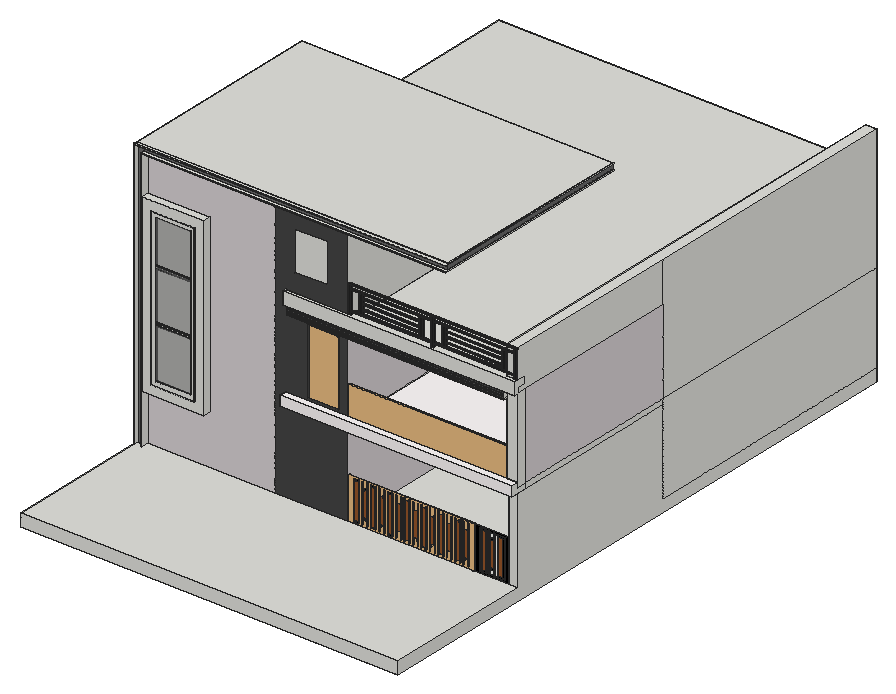
# SketchUp Ruby script. Lengths in inches.
U = 1.inch
M = Sketchup.active_model
def pt(a) = Geom::Point3d.new(a.map { |v| v * U })
def face(e, loops, mat)
  f = e.add_face(loops[0].map { |a| pt(a) })
  loops[1..].each { |l| e.add_face(l.map { |a| pt(a) }).erase! }
  f.material = f.back_material = mat if mat
  f
end
# faces: each face lists its corners as indices into pts; further lists are holes
def faces(e, pts, list, mat = nil) = list.each { |f| face(e, (f[0].is_a?(Array) ? f : [f]).map { |l| l.map { |i| pts[i] } }, mat) }
# xy, xz, yz: faces in a plane at the given z, y or x. An outline is a flat list of corners, or four numbers for a rectangle; further outlines are holes
def ring(l) = l.size == 4 ? [[l[0], l[1]], [l[2], l[1]], [l[2], l[3]], [l[0], l[3]]] : l.each_slice(2).to_a
def flat(e, list, mat, &to3) = list.each { |f| face(e, (f[0].is_a?(Array) ? f : [f]).map { |l| ring(l).map { |u, v| to3.(u, v) } }, mat) }
def xy(e, z, list, mat = nil) = flat(e, list, mat) { |x, y| [x, y, z] }
def xz(e, y, list, mat = nil) = flat(e, list, mat) { |x, z| [x, y, z] }
def yz(e, x, list, mat = nil) = flat(e, list, mat) { |y, z| [x, y, z] }
def lines(e, pts, list) = list.each { |a, b| e.add_line(pt(pts[a]), pt(pts[b])) }
# prism: a flat outline (further loops are holes) pulled along v
def prism(e, loops, v, mat = nil)
  f = face(e, loops, mat); d = Geom::Vector3d.new(v.map { |x| x * U })
  f.pushpull(f.normal.samedirection?(d) ? d.length : -d.length)
end
def box(e, o, s, mat = nil) = prism(e, [[o, [o[0] + s[0], o[1], o[2]], [o[0] + s[0], o[1] + s[1], o[2]], [o[0], o[1] + s[1], o[2]]]], [0, 0, s[2]], mat)
def at(x, y, z, deg = 0) = Geom::Transformation.translation(pt([x, y, z])) * Geom::Transformation.rotation(ORIGIN, Z_AXIS, deg.degrees)
def axes(o, x, y, z) = Geom::Transformation.new([*x, 0, *y, 0, *z, 0, *pt(o).to_a, 1])
def part(name) = M.definitions.add(name)
# library, detail: a bought-in or finely detailed component or shape, given as its bounding box
def library(name, o, s) = part(name).tap { |d| box(d.entities, o, s) }
def detail(e, o, s) = box(e.add_group.entities, o, s)
def put(e, d, t, mat = nil) = e.add_instance(d, t).tap { |i| i.material = mat if mat }
def group(e, t, mat = nil) = e.add_group.tap { |g| g.transformation = t; g.material = mat if mat }.entities
root = M.entities
M.materials.add("Painted Metal Railing").color = [35, 35, 35]
M.materials.add("[0010_Snow]").color = [255, 250, 250]
M.materials.add("[0134_DimGray]").color = [105, 105, 105]
M.materials.add("[0135_DarkGray]").color = [81, 81, 81]
M.materials.add("[Blinds Cellular White]").color = [217, 211, 213]
M.materials.add("[Blinds Cellular White]1").color = [217, 211, 213]
M.materials.add("[Blinds Wood Light]").color = [155, 100, 14]
M.materials.add("[Color M04]").color = [142, 142, 142]
M.materials.add("[Color M09]").color = [0, 0, 0]
M.materials.add("[Granite Dark Gray]").color = [69, 68, 68]
M.materials.add("[Translucent Glass Gray]").color = [128, 128, 128]
M.materials["[Translucent Glass Gray]"].alpha = 0.5
M.materials.add("[Wood Cherry Original]").color = [151, 86, 41]
M.materials.add("[Wood Veneer 01]").color = [119, 70, 35]
c1 = library("Untitled (14)",[0,0,0],[7.13,36,83])
c2 = library("Glass Railings(black Handrails)",[-57.04,-132.55,0],[169.29,2.52,28.17])
c3 = part("Post")
box(c3.entities,[-0.75,-0.75,0],[1.5,1.5,34.5],"Painted Metal Railing")
c4 = part("Group43\#1")
box(c4.entities,[-0.75,0,0],[1.5,73.5,1.5],"Painted Metal Railing")
c5 = part("Group46\#1")
box(c5.entities,[-0.75,0.75,0],[1.5,34.5,1.5],"Painted Metal Railing")
c6 = part("Group49\#1")
box(c6.entities,[-0.75,0.75,0],[1.5,34.5,1.5],"Painted Metal Railing")
c7 = part("Group52\#1")
box(c7.entities,[-0.75,0.75,0],[1.5,34.5,1.5],"Painted Metal Railing")
c8 = part("Group55\#1")
box(c8.entities,[-0.75,0.75,0],[1.5,34.5,1.5],"Painted Metal Railing")
c9 = part("Inner Post")
box(c9.entities,[-0.75,-0.75,0],[1.5,1.5,23.5],"Painted Metal Railing")
c10 = part("Group59\#1")
box(c10.entities,[-0.75,0.75,0],[1.5,24.5,1.5],"Painted Metal Railing")
c11 = part("Group62\#1")
box(c11.entities,[-0.75,0.75,0],[1.5,24.5,1.5],"Painted Metal Railing")
c12 = part("Group65\#1")
box(c12.entities,[-0.75,0.75,0],[1.5,24.5,1.5],"Painted Metal Railing")
c13 = part("Inner Posts and Rails\#2")
put(c13.entities,c9,at(0,0,0,90))
put(c13.entities,c9,at(0,26,0,90))
put(c13.entities,c10,at(0,0,4.75))
put(c13.entities,c11,at(0,0,11))
put(c13.entities,c12,at(0,0,17.25))
c14 = part("Group69\#1")
box(c14.entities,[-0.75,0.75,0],[1.5,24.5,1.5],"Painted Metal Railing")
c15 = part("Group72\#1")
box(c15.entities,[-0.75,0.75,0],[1.5,24.5,1.5],"Painted Metal Railing")
c16 = part("Group75\#1")
box(c16.entities,[-0.75,0.75,0],[1.5,24.5,1.5],"Painted Metal Railing")
c17 = part("Inner Posts and Rails\#3")
put(c17.entities,c9,at(0,0,0,90))
put(c17.entities,c9,at(0,26,0,90))
put(c17.entities,c14,at(0,0,4.75))
put(c17.entities,c15,at(0,0,11))
put(c17.entities,c16,at(0,0,17.25))
c18 = part("Railing Assembly 14\#1")
put(c18.entities,c3,at(0,0,0))
put(c18.entities,c3,at(36,0,0))
put(c18.entities,c3,at(72,0,0))
put(c18.entities,c4,at(-0.75,0,34.5,-90))
put(c18.entities,c5,at(0,0,4,-90))
put(c18.entities,c6,at(36,0,4,-90))
put(c18.entities,c7,at(0,0,29,-90))
put(c18.entities,c8,at(36,0,29,-90))
put(c18.entities,c13,at(5,0,5.5,-90))
put(c18.entities,c17,at(41,0,5.5,-90))
c19 = library("Decorative metal grille",[0,0,0],[271.62,130.55,3])
c20 = part("Group\#1")
xy(c20.entities,0,[[0.39,1.57,0.29,1.59,0.2,1.63,0.12,1.69,0.05,1.77,0.01,1.87,0,1.97,0.01,2.07,0.05,2.17,0.12,2.25,0.2,2.31,0.29,2.35,0.39,2.36,0.5,2.35,0.59,2.31,0.67,2.25,0.73,2.17,0.77,2.07,0.79,1.97,0.77,1.87,0.73,1.77,0.67,1.69,0.59,1.63,0.5,1.59],[0.39,13.39,0.29,13.4,0.2,13.4375,0.12,13.5,0.05,13.58,0.01,13.68,0,13.78,0.01,13.88,0.05,13.98,0.12,14.06,0.2,14.12,0.29,14.16,0.39,14.17,0.5,14.16,0.59,14.12,0.67,14.06,0.73,13.98,0.77,13.88,0.79,13.78,0.77,13.68,0.73,13.58,0.67,13.5,0.59,13.4375,0.5,13.4]])
xy(c20.entities,1.97,[[0.39,1.57,0.39,2.36,0.29,2.35,0.2,2.31,0.12,2.25,0.05,2.17,0.01,2.07,0,1.97,0.01,1.87,0.05,1.77,0.12,1.69,0.2,1.63,0.29,1.59],[0.39,1.57,0.5,1.59,0.59,1.63,0.67,1.69,0.73,1.77,0.77,1.87,0.79,1.97,0.77,2.07,0.73,2.17,0.67,2.25,0.59,2.31,0.5,2.35,0.39,2.36],[0.39,13.39,0.39,14.17,0.29,14.16,0.2,14.12,0.12,14.06,0.05,13.98,0.01,13.88,0,13.78,0.01,13.68,0.05,13.58,0.12,13.5,0.2,13.4375,0.29,13.4],[0.39,13.39,0.5,13.4,0.59,13.4375,0.67,13.5,0.73,13.58,0.77,13.68,0.79,13.78,0.77,13.88,0.73,13.98,0.67,14.06,0.59,14.12,0.5,14.16,0.39,14.17]])
xz(c20.entities,0,[[0.39,1.57,0.5,1.59,0.59,1.63,0.67,1.69,0.73,1.77,0.77,1.87,0.79,1.97,0.77,2.07,0.73,2.17,0.67,2.25,0.59,2.31,0.5,2.35,0.39,2.36,0.29,2.35,0.2,2.31,0.12,2.25,0.05,2.17,0.01,2.07,0,1.97,0.01,1.87,0.05,1.77,0.12,1.69,0.2,1.63,0.29,1.59]])
xz(c20.entities,15.75,[[0.39,1.57,0.29,1.59,0.2,1.63,0.12,1.69,0.05,1.77,0.01,1.87,0,1.97,0.01,2.07,0.05,2.17,0.12,2.25,0.2,2.31,0.29,2.35,0.39,2.36,0.5,2.35,0.59,2.31,0.67,2.25,0.73,2.17,0.77,2.07,0.79,1.97,0.77,1.87,0.73,1.77,0.67,1.69,0.59,1.63,0.5,1.59]])
p = [[0.12,1.69,0],[0.2,1.63,0],[0.2,1.63,1.63],[0.2,1.63,1.97],[0.12,1.69,1.97],[0.12,1.69,1.69],
  [0.29,1.59,0],[0.29,1.59,1.59],[0.29,1.59,1.97],[0.39,1.57,0],[0.39,1.57,1.57],[0.39,1.57,1.97],
  [0.5,1.59,0],[0.5,1.59,1.59],[0.5,1.59,1.97],[0.59,1.63,0],[0.59,1.63,1.63],[0.59,1.63,1.97],
  [0.67,1.69,0],[0.67,1.69,1.69],[0.67,1.69,1.97],[0.05,1.77,0],[0.05,1.77,1.97],[0.05,1.77,1.77],
  [0.73,1.77,0],[0.73,1.77,1.77],[0.73,1.77,1.97],[0.01,1.87,0],[0.01,1.87,1.97],[0.01,1.87,1.87],
  [0.77,1.87,0],[0.77,1.87,1.87],[0.77,1.87,1.97],[0,1.97,0],[0,1.97,1.97],[0.79,1.97,0],
  [0.79,1.97,1.97],[0.01,2.07,0],[0.01,2.07,1.97],[0.01,2.07,1.87],[0.77,2.07,0],[0.77,2.07,1.87],
  [0.77,2.07,1.97],[0.05,2.17,0],[0.05,2.17,1.97],[0.05,2.17,1.77],[0.73,2.17,0],[0.73,2.17,1.77],
  [0.73,2.17,1.97],[0.12,2.25,0],[0.12,2.25,1.97],[0.12,2.25,1.69],[0.2,2.31,0],[0.2,2.31,1.97],
  [0.2,2.31,1.63],[0.67,2.25,0],[0.59,2.31,0],[0.59,2.31,1.63],[0.59,2.31,1.97],[0.67,2.25,1.97],
  [0.67,2.25,1.69],[0.29,2.35,0],[0.29,2.35,1.97],[0.29,2.35,1.59],[0.39,2.36,0],[0.39,2.36,1.97],
  [0.39,2.36,1.57],[0.5,2.35,0],[0.5,2.35,1.97],[0.5,2.35,1.59],[0.12,13.5,0],[0.2,13.4375,0],
  [0.2,13.4375,1.63],[0.2,13.4375,1.97],[0.12,13.5,1.97],[0.12,13.5,1.69],[0.29,13.4,0],[0.29,13.4,1.59],
  [0.29,13.4,1.97],[0.39,13.39,0],[0.39,13.39,1.57],[0.39,13.39,1.97],[0.5,13.4,0],[0.5,13.4,1.59],
  [0.5,13.4,1.97],[0.59,13.4375,0],[0.59,13.4375,1.63],[0.59,13.4375,1.97],[0.67,13.5,0],[0.67,13.5,1.69],
  [0.67,13.5,1.97],[0.05,13.58,0],[0.05,13.58,1.97],[0.05,13.58,1.77],[0.73,13.58,0],[0.73,13.58,1.77],
  [0.73,13.58,1.97],[0.01,13.68,0],[0.01,13.68,1.97],[0.01,13.68,1.87],[0.77,13.68,0],[0.77,13.68,1.87],
  [0.77,13.68,1.97],[0,13.78,0],[0,13.78,1.97],[0.79,13.78,0],[0.79,13.78,1.97],[0.01,13.88,0],
  [0.01,13.88,1.97],[0.01,13.88,1.87],[0.77,13.88,0],[0.77,13.88,1.87],[0.77,13.88,1.97],[0.05,13.98,0],
  [0.05,13.98,1.97],[0.05,13.98,1.77],[0.73,13.98,0],[0.73,13.98,1.77],[0.73,13.98,1.97],[0.12,14.06,0],
  [0.12,14.06,1.97],[0.12,14.06,1.69],[0.67,14.06,0],[0.67,14.06,1.69],[0.67,14.06,1.97],[0.2,14.12,0],
  [0.2,14.12,1.97],[0.2,14.12,1.63],[0.29,14.16,0],[0.29,14.16,1.97],[0.29,14.16,1.59],[0.59,14.12,0],
  [0.5,14.16,0],[0.5,14.16,1.59],[0.5,14.16,1.97],[0.59,14.12,1.97],[0.59,14.12,1.63],[0.39,14.17,0],
  [0.39,14.17,1.97],[0.39,14.17,1.57],[0.12,15.75,1.69],[0.2,15.75,1.63],[0.2,0,1.63],[0.12,0,1.69],
  [0.29,15.75,1.59],[0.29,0,1.59],[0.39,15.75,1.57],[0.39,13.78,1.57],[0.39,1.97,1.57],[0.39,0,1.57],
  [0.5,15.75,1.59],[0.5,0,1.59],[0.59,15.75,1.63],[0.59,0,1.63],[0.67,15.75,1.69],[0.67,0,1.69],
  [0.05,15.75,1.77],[0.05,0,1.77],[0.73,15.75,1.77],[0.73,0,1.77],[0.01,15.75,1.87],[0.01,0,1.87],
  [0.77,15.75,1.87],[0.77,0,1.87],[0,15.75,1.97],[0,0,1.97],[0.79,15.75,1.97],[0.79,0,1.97],
  [0.01,15.75,2.07],[0.01,0,2.07],[0.77,15.75,2.07],[0.77,0,2.07],[0.05,15.75,2.17],[0.05,0,2.17],
  [0.73,15.75,2.17],[0.73,0,2.17],[0.12,15.75,2.25],[0.12,0,2.25],[0.2,15.75,2.31],[0.2,0,2.31],
  [0.67,15.75,2.25],[0.59,15.75,2.31],[0.59,0,2.31],[0.67,0,2.25],[0.29,15.75,2.35],[0.29,0,2.35],
  [0.39,15.75,2.36],[0.39,0,2.36],[0.5,15.75,2.35],[0.5,0,2.35],[0.39,1.97,1.97],[0.39,13.78,0],
  [0.39,1.97,0],[0.39,13.78,1.97],[0.39,0,1.97],[0.39,15.75,1.97]]
faces(c20.entities,p,[[0,1,2,3,4,5],[1,6,7,8,3,2],[6,9,10,11,8,7],[9,12,13,14,11,10],[12,15,16,17,14,13],[15,18,19,20,17,16],[21,0,5,4,22,23],[18,24,25,26,20,19],
  [27,21,23,22,28,29],[24,30,31,32,26,25],[33,27,29,28,34],[30,35,36,32,31],[37,33,34,38,39],[35,40,41,42,36],[43,37,39,38,44,45],[40,46,47,48,42,41],
  [49,43,45,44,50,51],[52,49,51,50,53,54],[55,56,57,58,59,60],[46,55,60,59,48,47],[61,52,54,53,62,63],[64,61,63,62,65,66],[67,64,66,65,68,69],[56,67,69,68,58,57],
  [70,71,72,73,74,75],[71,76,77,78,73,72],[76,79,80,81,78,77],[79,82,83,84,81,80],[82,85,86,87,84,83],[85,88,89,90,87,86],[91,70,75,74,92,93],[88,94,95,96,90,89],
  [97,91,93,92,98,99],[94,100,101,102,96,95],[103,97,99,98,104],[100,105,106,102,101],[107,103,104,108,109],[105,110,111,112,106],[113,107,109,108,114,115],[110,116,117,118,112,111],
  [119,113,115,114,120,121],[116,122,123,124,118,117],[125,119,121,120,126,127],[128,125,127,126,129,130],[131,132,133,134,135,136],[122,131,136,135,124,123],[137,128,130,129,138,139],[132,137,139,138,134,133],
  [140,141,127,72,54,2,142,143,5,51,75,121],[141,144,130,77,63,7,145,142,2,54,72,127],[144,146,139,147,80,66,148,10,149,145,7,63,77,130],[146,150,133,83,69,13,151,149,10,148,66,80,147,139],[150,152,136,86,57,16,153,151,13,69,83,133],[152,154,123,89,60,19,155,153,16,57,86,136],[156,140,121,75,51,5,143,157,23,45,93,115],[154,158,117,95,47,25,159,155,19,60,89,123],
  [160,156,115,93,45,23,157,161,29,39,99,109],[158,162,111,101,41,31,163,159,25,47,95,117],[164,160,109,99,39,29,161,165,34,104],[162,166,106,36,167,163,31,41,101,111],[168,164,104,34,165,169],[166,170,171,167,36,106],[172,168,169,173],[170,174,175,171],
  [176,172,173,177],[178,176,177,179],[180,181,182,183],[174,180,183,175],[184,178,179,185],[186,184,185,187],[188,186,187,189],[181,188,189,182]])
lines(c20.entities,p,[[190,148],[191,147],[148,192],[147,193],[11,194],[138,195],[81,65]])
c21 = part("3 80")
p = [[0,0,0],[1,0,0],[1,1,0]]
lines(c21.entities,p,[[0,1],[1,2],[2,0]])
g1 = group(c21.entities,at(0,0.01,-0.01))
g2 = group(g1,at(0,0,0))
xy(g2,0.01,[[0,-4.72,2.36,0],[33.86,-4.72,36.22,0],[2.36,-1.57,33.86,0]])
xy(g2,11.42,[[2.36,-1.97,33.86,-1.57]],"[Color M04]")
xy(g2,12.2,[[2.36,-1.97,33.86,-1.57]],"[Color M04]")
xy(g2,23.23,[[2.36,-1.97,33.86,-1.57]],"[Color M04]")
xy(g2,24.02,[[2.36,-1.97,33.86,-1.57]],"[Color M04]")
xy(g2,35.04,[[2.36,-1.97,33.86,-1.57]],"[Color M04]")
xy(g2,35.83,[[2.36,-1.97,33.86,-1.57]],"[Color M04]")
xy(g2,46.85,[[2.36,-2.36,33.86,-1.57]],"[Color M04]")
xy(g2,47.64,[[2.36,-2.36,33.86,-1.57]],"[Color M04]")
xy(g2,58.66,[[2.36,-2.36,33.86,-1.57]],"[Color M04]")
xy(g2,59.45,[[2.36,-2.36,33.86,-1.57]],"[Color M04]")
xy(g2,70.47,[[2.36,-2.36,33.86,-1.57]],"[Color M04]")
xy(g2,71.26,[[2.36,-2.36,33.86,-1.57]],"[Color M04]")
xy(g2,82.68,[[2.36,-4.72,33.86,-1.57]],"[Wood Veneer 01]")
xy(g2,85.04,[[0,-4.72,36.22,0]],"[Wood Veneer 01]")
xz(g2,-4.72,[[0,0.01,0,85.04,36.22,85.04,36.22,0.01,33.86,0.01,33.86,82.68,2.36,82.68,2.36,0.01]],"[Wood Veneer 01]")
xz(g2,-2.36,[[2.36,46.85,33.86,47.64],[2.36,58.66,33.86,59.45],[2.36,70.47,33.86,71.26]],"[Color M04]")
xz(g2,-1.97,[[2.36,11.42,33.86,12.2],[2.36,23.23,33.86,24.02],[2.36,35.04,33.86,35.83]],"[Color M04]")
xz(g2,-1.57,[[2.36,0.01,33.86,11.42],[2.36,12.2,33.86,23.23],[2.36,24.02,33.86,35.04],[2.36,35.83,33.86,46.85],[2.36,47.64,33.86,58.66],
  [2.36,59.45,33.86,70.47],[2.36,71.26,33.86,82.68]],"[Wood Veneer 01]")
xz(g2,0,[[0,0.01,2.36,0.01,2.36,82.68,33.86,82.68,33.86,0.01,36.22,0.01,36.22,85.04,0,85.04],[2.36,0.01,33.86,82.68]],"[Wood Veneer 01]")
yz(g2,0,[[-4.72,0.01,0,85.04]],"[Wood Veneer 01]")
yz(g2,2.36,[[-4.72,0.01,-4.72,82.68,-1.57,82.68,-1.57,71.26,-2.36,71.26,-2.36,70.47,-1.57,70.47,-1.57,59.45,-2.36,59.45,-2.36,58.66,-1.57,58.66,-1.57,47.64,-2.36,47.64,-2.36,46.85,-1.57,46.85,-1.57,35.83,-1.97,35.83,-1.97,35.04,-1.57,35.04,-1.57,24.02,-1.97,24.02,-1.97,23.23,-1.57,23.23,-1.57,12.2,-1.97,12.2,-1.97,11.42,-1.57,11.42,-1.57,0.01]],"[Wood Veneer 01]")
yz(g2,33.86,[[-4.72,0.01,-1.57,0.01,-1.57,11.42,-1.97,11.42,-1.97,12.2,-1.57,12.2,-1.57,23.23,-1.97,23.23,-1.97,24.02,-1.57,24.02,-1.57,35.04,-1.97,35.04,-1.97,35.83,-1.57,35.83,-1.57,46.85,-2.36,46.85,-2.36,47.64,-1.57,47.64,-1.57,58.66,-2.36,58.66,-2.36,59.45,-1.57,59.45,-1.57,70.47,-2.36,70.47,-2.36,71.26,-1.57,71.26,-1.57,82.68,-4.72,82.68]],"[Wood Veneer 01]")
yz(g2,36.22,[[-4.72,0.01,0,85.04]],"[Wood Veneer 01]")
p = [[0,0,0],[0,0,0.01]]
lines(g2,p,[[0,1]])
put(g1,c20,axes([30.98,0,38.01],[1,0,0],[0,0,1],[0,1,0]),"[Color M04]")
put(g1,c20,axes([30.98,-1.57,38.01],[1,0,0],[0,0,1],[0,-1,0]),"[Color M04]")
c22 = part("Window")
xy(c22.entities,0,[[0,0,19.69,1.97]])
xy(c22.entities,1.97,[[1.97,0,17.72,0.79]])
xy(c22.entities,1.97,[[1.97,0.79,17.72,1.97]],"[Translucent Glass Gray]")
xy(c22.entities,24.8,[[1.97,0,17.72,0.79]])
xy(c22.entities,24.8,[[1.97,0.79,17.72,1.97]],"[Translucent Glass Gray]")
xy(c22.entities,25.98,[[1.97,0,17.72,0.79],[1.97,0.79,17.72,1.97]])
xy(c22.entities,48.03,[[1.97,0,17.72,1.97]])
xy(c22.entities,49.21,[[1.97,0,17.72,0.79]])
xy(c22.entities,49.21,[[1.97,0.79,17.72,1.97]],"[Translucent Glass Gray]")
xy(c22.entities,68.9,[[1.97,0,17.72,0.79]])
xy(c22.entities,68.9,[[1.97,0.79,17.72,1.97]],"[Translucent Glass Gray]")
xy(c22.entities,70.87,[[0,0,19.69,1.97]])
xz(c22.entities,0,[[[0,0,19.69,70.87],[1.97,1.97,17.72,68.9]]])
xz(c22.entities,0.79,[[1.97,1.97,17.72,24.8],[1.97,25.98,17.72,48.82],[1.97,49.21,17.72,68.9]],"[Translucent Glass Gray]")
xz(c22.entities,1.97,[[[0,0,19.69,70.87],[1.97,1.97,17.72,68.9]],[1.97,24.8,17.72,25.98],[1.97,48.03,17.72,49.21]])
yz(c22.entities,0,[[0,0,1.97,70.87]])
yz(c22.entities,1.97,[[0,1.97,0.79,24.8],[0,24.8,1.97,25.98],[0,25.98,0.79,48.03],[0.79,25.98,1.97,48.03],[0,48.03,1.97,49.21],
  [0,49.21,0.79,68.9]])
yz(c22.entities,1.97,[[0.79,1.97,1.97,24.8],[0.79,49.21,1.97,68.9]],"[Translucent Glass Gray]")
yz(c22.entities,17.72,[[0,1.97,0.79,24.8],[0,24.8,1.97,25.98],[0,25.98,0.79,48.03],[0.79,25.98,1.97,48.03],[0,48.03,1.97,49.21],
  [0,49.21,0.79,68.9]])
yz(c22.entities,17.72,[[0.79,1.97,1.97,24.8],[0.79,49.21,1.97,68.9]],"[Translucent Glass Gray]")
yz(c22.entities,19.69,[[0,0,1.97,70.87]])
c23 = part("Group\#66")
box(c23.entities,[0,0,-0.39],[5.91,82.68,1.96])
c24 = part("Group\#67")
box(c24.entities,[0,0,-0.39],[5.91,118.11,1.96])
c25 = part("Group\#62")
box(c25.entities,[0,0,0],[5.91,5.91,1.18])
c26 = part("Group\#63")
box(c26.entities,[0,0,0],[5.91,5.91,1.18])
c27 = part("Group\#61")
prism(c27.entities,[[[0.98,124.02,0],[0.98,5.91,0],[0.98,0,0],[0,0,0],[0,129.92,0],[0.98,129.92,0]]],[0,0,1.18])
c28 = library("Group\#59",[0,0,0],[177.17,141.73,1.18])
c29 = part("Group\#64")
box(c29.entities,[0,0,0],[5.91,5.91,1.18])
c30 = part("Group\#65")
box(c30.entities,[0,0,0],[5.91,5.91,1.18])
xy(root,-16.125,[[0,0,505.375,800.5625]])
xy(root,0,[[0,0,505.375,0,505.375,200.5625,493.35,200.5625,493.35,443.4375,484.36,443.4375,484.36,504.8125,430.92,504.8125,430.92,443.4375,278.0625,443.4375,278.0625,200.5625,10,200.5625,10,190.5625,9,190.5625,9,195.5625,1,195.5625,1,190.5625,0,190.5625],[0,190.5625,1,195.5625],[9,190.5625,10,195.5625],[0,195.5625,10,195.5625,10,200.5625,278.0625,200.5625,278.0625,443.4375,430.92,443.4375,430.92,504.8125,484.36,504.8125,484.36,443.4375,505.375,443.4375,505.375,800.5625,0,800.5625]])
xy(root,66.03,[[10,190.5625,92.75,200.5625]])
xy(root,78.62,[[22.59,190.5625,80.16,200.5625]])
xy(root,108.5,[[430.92,443.4375,484.36,504.8125]],"[Blinds Cellular White]")
xy(root,113,[[195.125,190.6875,195.125,200.5625,278.0625,200.5625,278.0625,443.4375,493.35,443.4375,493.35,200.5625,505.375,200.5625,505.375,190.6875]],"[Blinds Wood Light]")
xy(root,120,[[490.93,200.0625,505.375,212.75]])
xy(root,120,[[278.0625,212.625,490.93,212.625,490.93,212.75,505.375,212.75,505.375,443.4375,278.0625,443.4375]],"[0010_Snow]")
xy(root,120,[[408.52,443.4375,471.83,456.625]],"[Blinds Cellular White]")
xy(root,126.5,[[195.125,190.6875,505.375,190.6875,505.375,200.0625,490.93,200.0625,490.93,212.625,278.0625,212.625,278.0625,200.5625,195.125,200.5625]],"[0010_Snow]")
xy(root,129.52,[[225.02,200.5625,265.77,208.875]],"[Granite Dark Gray]")
xy(root,218.01,[[225.02,200.5625,265.77,208.875]],"[Granite Dark Gray]")
xy(root,222.15,[[200.18,195.9375,490.93,200.0625]],"[0135_DarkGray]")
xy(root,222.44,[[408.52,443.4375,471.83,456.625]],"[Blinds Cellular White]")
xy(root,233,[[200.18,195.9375,490.93,200.0625],[200.18,200.5625,278.0625,212.75],[278.0625,200.5625,490.93,212.75],[490.93,200.5625,505.375,212.75]])
xy(root,233,[[195.125,195.25,195.125,200.5625,490.93,200.5625,490.93,200.0625,200.18,200.0625,200.18,195.9375,490.93,195.9375,490.93,200.0625,505.375,200.0625,505.375,195.25]],"[0135_DarkGray]")
xy(root,233,[[278.0625,212.75,505.375,443.4375]],"[Blinds Wood Light]")
xy(root,240,[[278.0625,200.5625,505.375,210.5],[278.0625,210.5,490.6875,210.5,490.6875,800.5625,0,800.5625,0,470.9375,278.0625,470.9375]])
xy(root,249,[[195.125,195.25,505.375,195.25,505.375,201.3125,490.6875,201.3125,490.6875,210.5,278.0625,210.5,278.0625,200.5625,195.125,200.5625],[490.6875,201.3125,505.375,210.5]])
xy(root,287.06,[[22.59,190.5625,80.16,200.5625]])
xy(root,287.16,[[490.6875,201.3125,505.375,800.5625]])
xy(root,299.65,[[10,190.5625,92.75,200.5625]])
xy(root,351,[[10,190.5625,180.375,195.5625],[180.375,190.5625,417.375,195.5625],[10,195.5625,180.375,200.5625],[180.375,195.5625,415.75,200.5625],[415.75,195.5625,417.37,470.9375],
  [278.0625,200.5625,415.75,470.9375]])
xy(root,352,[[9,190.5625,10,195.5625],[10,190.5625,417.375,195.5625],[415.75,195.5625,417.37,470.9375]])
xy(root,359,[[1,190.5625,1,195.5625,415.75,195.5625,415.75,470.9375,417.37,470.9375,417.37,190.5625]])
xy(root,360,[[0,190.5625,417.37,190.5625,417.37,470.9375,415.75,470.9375,415.75,195.5625,0,195.5625],[0,195.5625,415.75,470.9375]])
xz(root,0,[[0,-16.125,505.375,0]])
xz(root,190.5625,[[0,0,1,0,1,359,417.37,359,417.37,360,0,360],[9,0,10,0,10,351,417.375,351,417.375,352,9,352],[[10,66.03,92.75,299.65],[22.59,78.62,80.16,287.06]]])
xz(root,190.6875,[[195.125,113,505.375,126.5]],"[0010_Snow]")
xz(root,195.25,[[195.125,233,505.375,249]])
xz(root,195.5625,[[0,0,0,360,415.75,360,415.75,359,1,359,1,0],[280.57,351,415.75,352],[415.75,351,417.37,352],[417.37,351,417.375,352]])
xz(root,195.5625,[[1,0,9,0,9,352,415.75,352,415.75,359,1,359]],"[0134_DimGray]")
xz(root,195.9375,[[200.18,223.59,490.93,224.09],[200.18,226.26,490.93,227.0625],[200.18,229.23,490.93,230.03]])
xz(root,195.9375,[[200.18,222.15,490.93,223.59],[200.18,224.09,490.93,226.26],[200.18,227.0625,490.93,229.23],[200.18,230.03,490.93,233]],"[0135_DarkGray]")
xz(root,200.0625,[[490.93,120,505.375,126.5],[490.93,126.5,505.375,233],[200.18,222.15,490.93,224.09],[200.18,224.09,490.93,233]])
xz(root,200.5625,[[493.35,0,505.375,113],[22.59,78.62,80.16,287.06],[195.125,113,278.0625,126.5],[195.125,233,278.0625,249],[206.59,273.26,250.59,326.07]])
xz(root,200.5625,[[10,0,180.375,0,180.375,351,10,351,10,299.65,92.75,299.65,92.75,66.03,10,66.03]],"[Blinds Cellular White]1")
xz(root,200.5625,[[[180.375,0,278.0625,0,278.0625,113,195.125,113,195.125,126.5,278.0625,126.5,278.0625,233,195.125,233,195.125,249,278.0625,249,278.0625,351,180.375,351],[225.02,129.52,265.77,218.01],[206.59,273.26,250.59,326.07]]],"[Granite Dark Gray]")
xz(root,201.3125,[[490.6875,249,505.375,287.16]])
xz(root,208.875,[[225.02,129.52,265.77,218.01]],"[Granite Dark Gray]")
xz(root,210.5,[[278.0625,240,490.6875,249],[490.6875,240,505.375,249]])
xz(root,212.625,[[278.0625,120,490.93,126.5]])
xz(root,212.75,[[490.93,120,505.375,233],[200.18,224.09,490.93,233]])
xz(root,443.4375,[[493.35,0,505.375,113],[278.0625,113,505.375,120]])
xz(root,443.4375,[[278.0625,0,430.92,0,430.92,108.5,484.36,108.5,484.36,0,493.35,0,493.35,113,278.0625,113],[278.0625,120,408.52,120,408.52,222.44,471.83,222.44,471.83,120,505.375,120,505.375,233,278.0625,233]],"[Blinds Cellular White]")
xz(root,456.625,[[408.52,120,471.83,222.44]],"[Blinds Cellular White]")
xz(root,470.9375,[[0,240,0,360,415.75,360,415.75,351,278.0625,351,278.0625,240],[415.75,351,417.37,352],[415.75,359,417.37,360]])
xz(root,504.8125,[[430.92,0,484.36,108.5]],"[Blinds Cellular White]")
xz(root,800.5625,[[0,-16.125,505.375,0],[0,0,505.375,120],[0,120,0,240,490.6875,240,490.6875,287.16,505.375,287.16,505.375,120]])
yz(root,0,[[0,-16.125,800.5625,0],[190.5625,0,195.5625,120],[195.5625,0,800.5625,120],[190.5625,120,195.5625,240],[195.5625,120,800.5625,240],
  [190.5625,240,195.5625,360],[195.5625,240,470.9375,360]])
yz(root,1,[[190.5625,0,195.5625,359]])
yz(root,9,[[190.5625,0,195.5625,351],[190.5625,351,195.5625,352]])
yz(root,10,[[190.5625,0,200.5625,66.03],[190.5625,299.65,200.5625,351]])
yz(root,22.59,[[190.5625,78.62,200.5625,287.06]])
yz(root,80.16,[[190.5625,78.62,200.5625,287.06]])
yz(root,92.75,[[190.5625,66.03,200.5625,299.65]])
yz(root,195.125,[[190.6875,113,200.5625,126.5],[195.25,233,200.5625,249]])
yz(root,200.18,[[195.9375,222.15,200.0625,233]],"[0135_DarkGray]")
yz(root,225.02,[[200.5625,129.52,208.875,218.01]],"[Granite Dark Gray]")
yz(root,265.77,[[200.5625,129.52,208.875,218.01]],"[Granite Dark Gray]")
yz(root,278.0625,[[200.5625,113,443.4375,120],[200.5625,120,212.625,126.5],[200.5625,233,443.4375,240],[200.5625,240,210.5,249],[210.5,240,470.9375,240,470.9375,351,200.5625,351,200.5625,249,210.5,249]])
yz(root,278.0625,[[200.5625,0,443.4375,113],[212.625,120,443.4375,120,443.4375,233,200.5625,233,200.5625,126.5,212.625,126.5]],"[Blinds Cellular White]")
yz(root,408.52,[[443.4375,120,456.625,222.44]],"[Blinds Cellular White]")
yz(root,415.75,[[195.5625,351,470.9375,352],[195.5625,359,470.9375,360]])
yz(root,415.75,[[195.5625,352,470.9375,359]],"[0134_DimGray]")
yz(root,417.37,[[195.5625,351,470.9375,352],[190.5625,359,470.9375,360]])
yz(root,417.375,[[190.5625,351,195.5625,352]])
yz(root,430.92,[[443.4375,0,504.8125,108.5]],"[Blinds Cellular White]")
yz(root,471.83,[[443.4375,120,456.625,222.44]],"[Blinds Cellular White]")
yz(root,484.36,[[443.4375,0,504.8125,108.5]],"[Blinds Cellular White]")
yz(root,490.6875,[[210.5,240,210.5,249,201.3125,249,201.3125,287.16,219.25,287.16,219.25,240],[219.25,240,443.4375,287.16],[443.4375,240,800.5625,287.16]])
yz(root,490.93,[[200.0625,120,212.625,126.5],[212.625,120,212.625,126.5,200.0625,126.5,200.0625,224.09,212.75,224.09,212.75,120],[195.9375,222.15,200.0625,224.09],[195.9375,224.09,200.0625,233],[200.0625,224.09,212.75,233]])
yz(root,493.35,[[200.5625,0,443.4375,113]],"[Blinds Cellular White]")
yz(root,505.375,[[0,-16.125,800.5625,-16.125,800.5625,0,443.4375,0,443.4375,113,200.5625,113,200.5625,0,0,0],[443.4375,0,800.5625,120],[190.6875,113,212.75,113,212.75,120,200.0625,120,200.0625,126.5,190.6875,126.5],[212.75,113,443.4375,120],[200.0625,120,212.75,120,212.75,233,200.5625,233,200.5625,240,210.5,240,210.5,249,195.25,249,195.25,233,200.0625,233],
  [443.4375,120,800.5625,287.16],[200.5625,233,443.4375,233,443.4375,287.16,201.3125,287.16,201.3125,249,210.5,249,210.5,240,200.5625,240]])
yz(root,505.375,[[212.75,120,443.4375,233]],"[Blinds Cellular White]")
p = [[-387.79,-728.5,0],[-371.98,-728.5,0]]
lines(root,p,[[0,1]])
put(root,c1,axes([471.83,443.4375,120],[0,1,0],[-1.76,0,0],[0,0,1.23424]))
put(root,c2,axes([349.5,333.11,126.5],[1.26,0,0],[0,1,0],[0,0,1.37]))
put(root,c18,axes([280.38,200.5625,249],[3.09269,0,0],[0,1,0],[0,0,1.06]))
put(root,c19,axes([265.77,200.63,216.95],[0,0,-0.3219],[-0.31215,0,0],[0,0.29,0]))
put(root,c21,axes([430.92,448.15,0],[1.48,0,0],[0,1,0],[0,0,1.27598]))
put(root,c22,axes([22.59,190.5625,78.62],[3,0,0],[0,1,0],[0,0,2.94128]))
g3 = group(root,at(278.0625,200.5625,0),"[Color M09]")
g4 = group(g3,at(8.46,0,4.72),"[Wood Cherry Original]")
put(g4,c23,axes([11.28,0.63,7.09],[0.95518,0,0],[0,0,0.4],[0,-0.4,0]))
put(g4,c24,axes([192.73,0.63,0],[0.95518,0,0],[0,0,0.4],[0,-0.4,0]))
put(g4,c24,axes([170.17,0.63,0],[0.95518,0,0],[0,0,0.4],[0,-0.4,0]))
put(g4,c24,axes([22.5625,0.63,0],[0.95518,0,0],[0,0,0.4],[0,-0.4,0]))
put(g4,c24,axes([0,0.63,0],[0.95518,0,0],[0,0,0.4],[0,-0.4,0]))
put(g4,c23,axes([124.1,0.63,7.09],[0.95518,0,0],[0,0,0.4],[0,-0.4,0]))
put(g4,c23,axes([33.85,0.63,7.09],[0.95518,0,0],[0,0,0.4],[0,-0.4,0]))
put(g4,c24,axes([112.82,0.63,0],[0.95518,0,0],[0,0,0.4],[0,-0.4,0]))
put(g4,c23,axes([181.45,0.63,7.09],[0.95518,0,0],[0,0,0.4],[0,-0.4,0]))
put(g4,c24,axes([90.25,0.63,0],[0.95518,0,0],[0,0,0.4],[0,-0.4,0]))
put(g4,c23,axes([78.97,0.63,7.09],[0.95518,0,0],[0,0,0.4],[0,-0.4,0]))
put(g4,c23,axes([101.54,0.63,7.09],[0.95518,0,0],[0,0,0.4],[0,-0.4,0]))
put(g4,c24,axes([45.125,0.63,0],[0.95518,0,0],[0,0,0.4],[0,-0.4,0]))
put(g4,c24,axes([135.38,0.63,0],[0.95518,0,0],[0,0,0.4],[0,-0.4,0]))
put(g4,c23,axes([146.66,0.63,7.09],[0.95518,0,0],[0,0,0.4],[0,-0.4,0]))
put(g4,c23,axes([56.41,0.63,7.09],[0.95518,0,0],[0,0,0.4],[0,-0.4,0]))
put(g4,c24,axes([67.69,0.63,0],[0.95518,0,0],[0,0,0.4],[0,-0.4,0]))
g5 = group(g3,at(0,0.16,0))
put(g5,c25,axes([31.02,0.47,2.36],[0.95518,0,0],[0,0,0.4],[0,-0.4,0]))
put(g5,c26,axes([31.02,0.47,51.97],[0.95518,0,0],[0,0,0.4],[0,-0.4,0]))
g6 = group(g5,at(0,0.47,0))
put(g6,c27,axes([47.95,0,2.36],[0.95518,0,0],[0,0,0.4],[0,-0.4,0]))
put(g6,c27,axes([25.38,0,2.36],[0.95518,0,0],[0,0,0.4],[0,-0.4,0]))
put(g6,c27,axes([14.1,0,2.36],[0.95518,0,0],[0,0,0.4],[0,-0.4,0]))
put(g6,c27,axes([52.65,0,2.36],[0.95518,0,0],[0,0,0.4],[0,-0.4,0]))
put(g6,c27,axes([18.8,0,2.36],[0.95518,0,0],[0,0,0.4],[0,-0.4,0]))
put(g6,c27,axes([41.37,0,2.36],[0.95518,0,0],[0,0,0.4],[0,-0.4,0]))
put(g6,c27,axes([81.79,0,2.36],[0.95518,0,0],[0,0,0.4],[0,-0.4,0]))
put(g6,c27,axes([86.49,0,2.36],[0.95518,0,0],[0,0,0.4],[0,-0.4,0]))
put(g6,c27,axes([138.2,0,2.36],[0.95518,0,0],[0,0,0.4],[0,-0.4,0]))
put(g6,c27,axes([70.51,0,2.36],[0.95518,0,0],[0,0,0.4],[0,-0.4,0]))
put(g6,c27,axes([75.21,0,2.36],[0.95518,0,0],[0,0,0.4],[0,-0.4,0]))
put(g6,c27,axes([120.34,0,2.36],[0.95518,0,0],[0,0,0.4],[0,-0.4,0]))
put(g6,c27,axes([149.48,0,2.36],[0.95518,0,0],[0,0,0.4],[0,-0.4,0]))
put(g6,c27,axes([160.76,0,2.36],[0.95518,0,0],[0,0,0.4],[0,-0.4,0]))
put(g6,c27,axes([59.23,0,2.36],[0.95518,0,0],[0,0,0.4],[0,-0.4,0]))
put(g6,c27,axes([154.18,0,2.36],[0.95518,0,0],[0,0,0.4],[0,-0.4,0]))
put(g6,c27,axes([104.36,0,2.36],[0.95518,0,0],[0,0,0.4],[0,-0.4,0]))
put(g6,c27,axes([30.08,0,2.36],[0.95518,0,0],[0,0,0.4],[0,-0.4,0]))
put(g6,c27,axes([93.07,0,2.36],[0.95518,0,0],[0,0,0.4],[0,-0.4,0]))
put(g6,c27,axes([131.62,0,2.36],[0.95518,0,0],[0,0,0.4],[0,-0.4,0]))
put(g6,c27,axes([63.93,0,2.36],[0.95518,0,0],[0,0,0.4],[0,-0.4,0]))
put(g6,c27,axes([109.06,0,2.36],[0.95518,0,0],[0,0,0.4],[0,-0.4,0]))
put(g6,c27,axes([36.67,0,2.36],[0.95518,0,0],[0,0,0.4],[0,-0.4,0]))
put(g6,c27,axes([126.92,0,2.36],[0.95518,0,0],[0,0,0.4],[0,-0.4,0]))
put(g6,c27,axes([115.64,0,2.36],[0.95518,0,0],[0,0,0.4],[0,-0.4,0]))
put(g6,c27,axes([97.77,0,2.36],[0.95518,0,0],[0,0,0.4],[0,-0.4,0]))
put(g6,c28,axes([0,0,0],[0.95518,0,0],[0,0,0.4],[0,-0.4,0]))
g7 = group(g6,at(170.17,0,0))
prism(g7,[[[45.125,-0.47,56.69],[0,-0.47,56.69],[0,-0.47,0],[45.125,-0.47,0]],[[18.8,-0.47,54.33],[19.74,-0.47,54.33],[25.38,-0.47,54.33],[26.32,-0.47,54.33],[30.08,-0.47,54.33],[31.02,-0.47,54.33],[36.67,-0.47,54.33],[37.61,-0.47,54.33],[39.49,-0.47,54.33],[39.49,-0.47,2.36],[37.61,-0.47,2.36],[36.67,-0.47,2.36],[31.02,-0.47,2.36],[30.08,-0.47,2.36],[26.32,-0.47,2.36],[25.38,-0.47,2.36],[19.74,-0.47,2.36],[18.8,-0.47,2.36],[15.04,-0.47,2.36],[14.1,-0.47,2.36],[8.46,-0.47,2.36],[7.52,-0.47,2.36],[5.64,-0.47,2.36],[5.64,-0.47,54.33],[7.52,-0.47,54.33],[8.46,-0.47,54.33],[14.1,-0.47,54.33],[15.04,-0.47,54.33]]],[0,0.47,0])
put(g6,c27,axes([7.52,0,2.36],[0.95518,0,0],[0,0,0.4],[0,-0.4,0]))
put(g6,c27,axes([177.6875,0,2.36],[0.95518,0,0],[0,0,0.4],[0,-0.4,0]))
put(g6,c27,axes([206.83,0,2.36],[0.95518,0,0],[0,0,0.4],[0,-0.4,0]))
put(g6,c27,axes([195.55,0,2.36],[0.95518,0,0],[0,0,0.4],[0,-0.4,0]))
put(g6,c27,axes([188.97,0,2.36],[0.95518,0,0],[0,0,0.4],[0,-0.4,0]))
put(g6,c27,axes([184.27,0,2.36],[0.95518,0,0],[0,0,0.4],[0,-0.4,0]))
put(g6,c27,axes([200.25,0,2.36],[0.95518,0,0],[0,0,0.4],[0,-0.4,0]))
put(g6,c27,axes([142.9,0,2.36],[0.95518,0,0],[0,0,0.4],[0,-0.4,0]))
put(g5,c26,axes([143.84,0.47,51.97],[0.95518,0,0],[0,0,0.4],[0,-0.4,0]))
put(g5,c25,axes([201.19,0.47,2.36],[0.95518,0,0],[0,0,0.4],[0,-0.4,0]))
put(g5,c26,axes([98.71,0.47,51.97],[0.95518,0,0],[0,0,0.4],[0,-0.4,0]))
put(g5,c29,axes([189.91,0.47,44.88],[0.95518,0,0],[0,0,0.4],[0,-0.4,0]))
put(g5,c29,axes([42.31,0.47,44.88],[0.95518,0,0],[0,0,0.4],[0,-0.4,0]))
put(g5,c26,axes([178.625,0.47,51.97],[0.95518,0,0],[0,0,0.4],[0,-0.4,0]))
put(g5,c30,axes([87.43,0.47,9.45],[0.95518,0,0],[0,0,0.4],[0,-0.4,0]))
put(g5,c30,axes([155.125,0.47,9.45],[0.95518,0,0],[0,0,0.4],[0,-0.4,0]))
put(g5,c30,axes([110,0.47,9.45],[0.95518,0,0],[0,0,0.4],[0,-0.4,0]))
put(g5,c30,axes([42.31,0.47,9.45],[0.95518,0,0],[0,0,0.4],[0,-0.4,0]))
put(g5,c25,axes([178.625,0.47,2.36],[0.95518,0,0],[0,0,0.4],[0,-0.4,0]))
put(g5,c25,axes([8.46,0.47,2.36],[0.95518,0,0],[0,0,0.4],[0,-0.4,0]))
put(g5,c29,axes([19.74,0.47,44.88],[0.95518,0,0],[0,0,0.4],[0,-0.4,0]))
put(g5,c26,axes([8.46,0.47,51.97],[0.95518,0,0],[0,0,0.4],[0,-0.4,0]))
put(g5,c30,axes([19.74,0.47,9.45],[0.95518,0,0],[0,0,0.4],[0,-0.4,0]))
put(g5,c29,axes([64.87,0.47,44.88],[0.95518,0,0],[0,0,0.4],[0,-0.4,0]))
put(g5,c30,axes([64.87,0.47,9.45],[0.95518,0,0],[0,0,0.4],[0,-0.4,0]))
put(g5,c30,axes([132.56,0.47,9.45],[0.95518,0,0],[0,0,0.4],[0,-0.4,0]))
put(g5,c25,axes([121.28,0.47,2.36],[0.95518,0,0],[0,0,0.4],[0,-0.4,0]))
put(g5,c26,axes([53.59,0.47,51.97],[0.95518,0,0],[0,0,0.4],[0,-0.4,0]))
put(g5,c25,axes([98.71,0.47,2.36],[0.95518,0,0],[0,0,0.4],[0,-0.4,0]))
put(g5,c26,axes([121.28,0.47,51.97],[0.95518,0,0],[0,0,0.4],[0,-0.4,0]))
put(g5,c29,axes([132.56,0.47,44.88],[0.95518,0,0],[0,0,0.4],[0,-0.4,0]))
put(g5,c26,axes([201.19,0.47,51.97],[0.95518,0,0],[0,0,0.4],[0,-0.4,0]))
put(g5,c30,axes([189.91,0.47,9.45],[0.95518,0,0],[0,0,0.4],[0,-0.4,0]))
put(g5,c29,axes([87.43,0.47,44.88],[0.95518,0,0],[0,0,0.4],[0,-0.4,0]))
put(g5,c25,axes([143.84,0.47,2.36],[0.95518,0,0],[0,0,0.4],[0,-0.4,0]))
put(g5,c25,axes([53.59,0.47,2.36],[0.95518,0,0],[0,0,0.4],[0,-0.4,0]))
put(g5,c29,axes([155.125,0.47,44.88],[0.95518,0,0],[0,0,0.4],[0,-0.4,0]))
put(g5,c25,axes([76.15,0.47,2.36],[0.95518,0,0],[0,0,0.4],[0,-0.4,0]))
put(g5,c26,axes([76.15,0.47,51.97],[0.95518,0,0],[0,0,0.4],[0,-0.4,0]))
put(g5,c29,axes([110,0.47,44.88],[0.95518,0,0],[0,0,0.4],[0,-0.4,0]))
